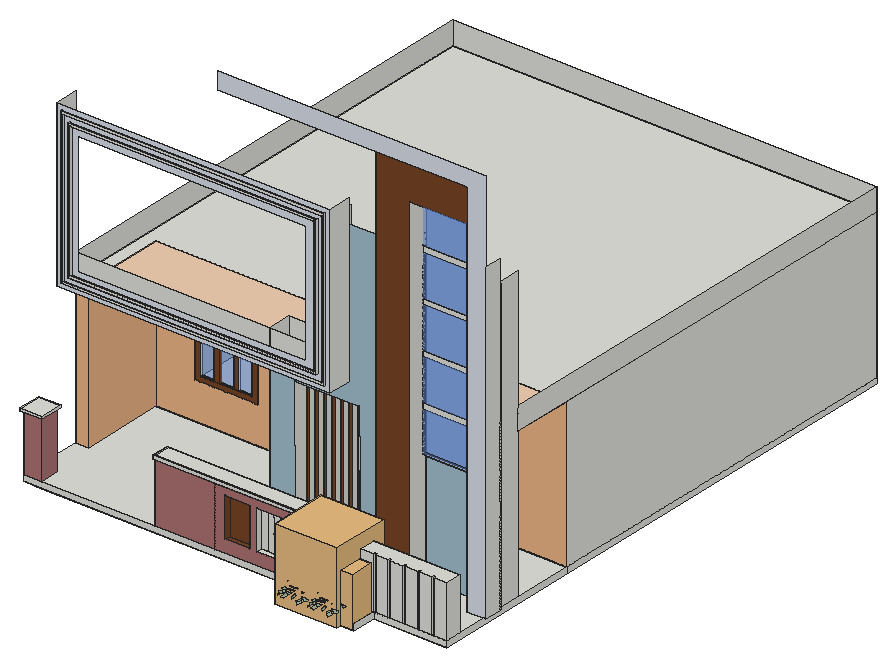
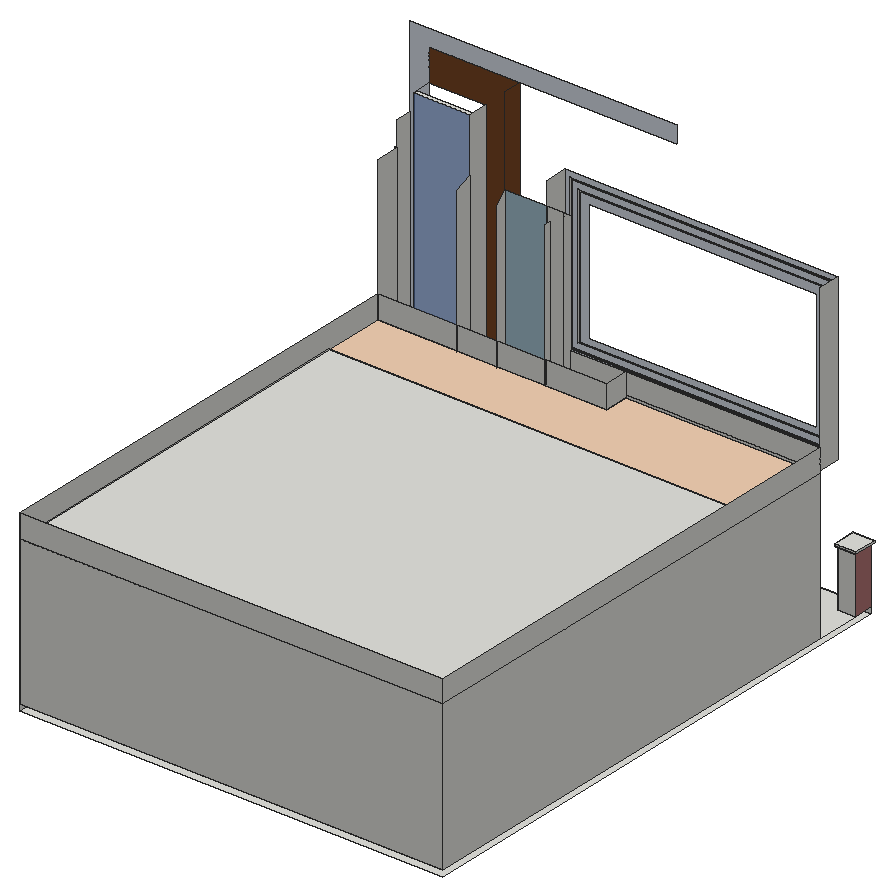
# SketchUp Ruby script. Lengths in inches.
U = 1.inch
M = Sketchup.active_model
def pt(a) = Geom::Point3d.new(a.map { |v| v * U })
def face(e, loops, mat)
  f = e.add_face(loops[0].map { |a| pt(a) })
  loops[1..].each { |l| e.add_face(l.map { |a| pt(a) }).erase! }
  f.material = f.back_material = mat if mat
  f
end
# faces: each face lists its corners as indices into pts; further lists are holes
def faces(e, pts, list, mat = nil) = list.each { |f| face(e, (f[0].is_a?(Array) ? f : [f]).map { |l| l.map { |i| pts[i] } }, mat) }
# xy, xz, yz: faces in a plane at the given z, y or x. An outline is a flat list of corners, or four numbers for a rectangle; further outlines are holes
def ring(l) = l.size == 4 ? [[l[0], l[1]], [l[2], l[1]], [l[2], l[3]], [l[0], l[3]]] : l.each_slice(2).to_a
def flat(e, list, mat, &to3) = list.each { |f| face(e, (f[0].is_a?(Array) ? f : [f]).map { |l| ring(l).map { |u, v| to3.(u, v) } }, mat) }
def xy(e, z, list, mat = nil) = flat(e, list, mat) { |x, y| [x, y, z] }
def xz(e, y, list, mat = nil) = flat(e, list, mat) { |x, z| [x, y, z] }
def yz(e, x, list, mat = nil) = flat(e, list, mat) { |y, z| [x, y, z] }
def lines(e, pts, list) = list.each { |a, b| e.add_line(pt(pts[a]), pt(pts[b])) }
# prism: a flat outline (further loops are holes) pulled along v
def prism(e, loops, v, mat = nil)
  f = face(e, loops, mat); d = Geom::Vector3d.new(v.map { |x| x * U })
  f.pushpull(f.normal.samedirection?(d) ? d.length : -d.length)
end
def box(e, o, s, mat = nil) = prism(e, [[o, [o[0] + s[0], o[1], o[2]], [o[0] + s[0], o[1] + s[1], o[2]], [o[0], o[1] + s[1], o[2]]]], [0, 0, s[2]], mat)
def at(x, y, z, deg = 0) = Geom::Transformation.translation(pt([x, y, z])) * Geom::Transformation.rotation(ORIGIN, Z_AXIS, deg.degrees)
def axes(o, x, y, z) = Geom::Transformation.new([*x, 0, *y, 0, *z, 0, *pt(o).to_a, 1])
def part(name) = M.definitions.add(name)
# library, detail: a bought-in or finely detailed component or shape, given as its bounding box
def library(name, o, s) = part(name).tap { |d| box(d.entities, o, s) }
def detail(e, o, s) = box(e.add_group.entities, o, s)
def put(e, d, t, mat = nil) = e.add_instance(d, t).tap { |i| i.material = mat if mat }
def group(e, t, mat = nil) = e.add_group.tap { |g| g.transformation = t; g.material = mat if mat }.entities
root = M.entities
M.materials.add("Generic").color = [175, 116, 116]
M.materials.add("Generic\#1").color = [243, 208, 179]
M.materials.add("Generic\#2").color = [164, 192, 208]
M.materials.add("Generic\#3").color = [219, 225, 235]
M.materials.add("Generic\#4").color = [240, 183, 136]
M.materials.add("[Translucent Glass Blue]").color = [100, 149, 237]
M.materials["[Translucent Glass Blue]"].alpha = 0.5
M.materials.add("[Wood Veneer 01]").color = [120, 70, 37]
M.materials.add("hymenocallis littoralis").color = [156, 172, 146]
c1 = part("Group\#856")
xy(c1.entities,7.38,[[0,0,5.5,15.91]],"hymenocallis littoralis")
p = [[5.5,28.78,0],[5.5,26.79,3.44],[0,26.79,3.44],[0,28.78,0],[0,23.75,6],[5.5,23.75,6],
  [0,15.91,7.38],[5.5,15.91,7.38]]
faces(c1.entities,p,[[0,1,2,3],[4,2,1,5],[6,4,5,7]],"hymenocallis littoralis")
c2 = part("Group\#854")
xy(c2.entities,7.38,[[0,0,5.5,15.91],[0,15.91,5.5,23.87]],"hymenocallis littoralis")
p = [[5.5,31.07,4.3],[5.5,27.74,6.47],[0,27.74,6.47],[0,31.07,4.3],[0,23.87,7.38],[5.5,23.87,7.38]]
faces(c2.entities,p,[[0,1,2,3],[4,2,1,5]],"hymenocallis littoralis")
c3 = part("Group\#857")
xy(c3.entities,7.38,[[0,0,5.6,15.91]],"hymenocallis littoralis")
p = [[5.6,28.78,0],[5.6,26.79,3.44],[0,26.79,3.44],[0,28.78,0],[0,23.75,6],[5.6,23.75,6],
  [0,15.91,7.38],[5.6,15.91,7.38]]
faces(c3.entities,p,[[0,1,2,3],[4,2,1,5],[6,4,5,7]],"hymenocallis littoralis")
c4 = part("Group\#855")
put(c4.entities,c2,axes([6.09,8.57,-0.52],[0.446,0.85617,0.26089],[-0.18444,-0.19731,0.96283],[0.87582,-0.47754,0.0699]))
put(c4.entities,c2,axes([6.29,7.28,-1.71],[0.37058,0.92707,-0.05667],[-0.32382,0.19004,0.99128],[0.87712,-0.32925,0.34964]))
put(c4.entities,c2,axes([11.04,16.14,-0.7],[1,0,0],[0,0.16628,1.02662],[0,-1.18456,0.19186]))
c5 = part("Group\#860")
put(c5.entities,c1,axes([24.57,32.05,-1.76],[0.9552,-0.22102,-0.19681],[0.4036,0.95545,0.88585],[-0.00568,-0.67859,0.7345]))
put(c5.entities,c1,axes([23.95,29.24,-2.4],[0,1,0],[-0.76041,0,0.64945],[0.64945,0,0.76041]))
put(c5.entities,c1,axes([24.22,24.72,-0.48],[-0.70711,0.70711,0],[-0.32757,-0.32757,0.80237],[0.61237,0.61237,0.5]))
put(c5.entities,c2,axes([20.66,37.22,-0.63],[1.12361,0.03262,0.39091],[-0.43499,0.29739,0.78777],[0.09852,-1.27434,0.37535]))
put(c5.entities,c1,axes([28.75,24.45,-2.4],[-1,0,0],[0,-0.76041,0.64945],[0,0.64945,0.76041]))
put(c5.entities,c3,axes([30.4,30.98,-3.7],[0.65676,-0.72002,0.22414],[0.55667,0.66341,0.5],[-0.50871,-0.20361,0.83652]))
put(c5.entities,c3,axes([32.41,29.61,-3.7],[0.04029,-0.97372,0.22414],[0.85287,0.15038,0.5],[-0.52057,0.17102,0.83652]))
put(c5.entities,c1,axes([31.89,25.85,-1.76],[-0.92056,0.33739,-0.19681],[-0.5186,-0.89824,0.88585],[0.08952,0.67268,0.7345]))
put(c5.entities,c1,axes([25.55,34.78,-0.48],[0.86603,0.5,0],[-0.25,0.43301,0.86603],[0.43301,-0.75,0.5]))
put(c5.entities,c3,axes([20.4,16.9375,-8.07],[-0.70711,0.70711,0],[-0.35754,-0.35754,0.65422],[1.3987,1.3987,1.52882]))
put(c5.entities,c1,axes([32.86,34.14,-0.48],[0.76604,-0.64279,0],[0.32139,0.38302,0.86603],[-0.55667,-0.66341,0.5]))
put(c5.entities,c1,axes([27.15,34.7,-0.1],[0.82472,-0.17528,-0.53769],[0.53769,0.53769,0.64945],[0.17528,-0.82472,0.53769]))
put(c5.entities,c1,axes([33.58,28.77,-2.4],[0,-1,0],[0.76041,0,0.64945],[-0.64945,0,0.76041]))
put(c5.entities,c1,axes([26.43,23.87,-2.81],[-0.75126,0.04415,0.65853],[0.53769,-0.53769,0.64945],[0.38276,0.84199,0.3802]))
put(c5.entities,c1,axes([28.78,23.98,-2.4],[-1,0,0],[0,-0.76041,0.64945],[0,0.64945,0.76041]))
put(c5.entities,c1,axes([25.39,25.38,-2.4],[-0.70711,0.70711,0],[-0.53769,-0.53769,0.64945],[0.45923,0.45923,0.76041]))
put(c5.entities,c1,axes([27.32,21.63,-0.1],[-0.45923,0.70711,-0.53769],[-0.76041,0,0.64945],[0.45923,0.70711,0.53769]))
put(c5.entities,c1,axes([25.17,27.625,-1.76],[0.56416,0.80187,-0.19681],[-0.66673,0.66673,0.80532],[0.62659,-0.26057,0.7345]))
put(c5.entities,c3,axes([27.59,27.04,-3.96],[-0.8993,-0.06127,0.43301],[0.2962,-0.8138,0.5],[0.32175,0.57791,0.75]))
put(c5.entities,c3,axes([26.98,24.5,-3.18],[-0.5,0.86603,0],[-0.75,-0.43301,0.5],[0.43301,0.25,0.86603]))
put(c5.entities,c3,axes([24.55,27.74,-3.7],[0.29517,0.92878,0.22414],[-0.85287,0.15038,0.5],[0.43068,-0.33875,0.83652]))
put(c5.entities,c3,axes([24.26,29.8,-3.18],[0.76604,0.64279,0],[-0.47317,0.5639,0.425],[0.32139,-0.38302,0.86603]))
put(c5.entities,c3,axes([25.98,32.46,-3.18],[1,0,0],[0,0.86603,0.5],[0,-0.5,0.86603]))
put(c5.entities,c1,axes([28.78,33.57,-2.4],[1,0,0],[0,0.76041,0.64945],[0,-0.64945,0.76041]))
put(c5.entities,c4,at(14.99,21.38,2.5))
put(c5.entities,c2,axes([34.63,26.34,-1.46],[-0.70089,-0.70877,0.07994],[0.4756,-0.38088,0.79293],[-0.53156,0.59378,0.60405]))
put(c5.entities,c2,axes([28.14,16.92,1.8125],[-1.19719,0.6912,0],[-0.09607,-0.16641,0.94244],[0.68444,1.18549,0.17613]))
put(c5.entities,c2,axes([31.5625,35.84,0.97],[0.66765,-1.1564,0.35779],[0.04445,0.30732,0.91033],[-1.20828,-0.64496,0.17012]))
put(c5.entities,c2,axes([38.94,22.51,0.89],[-0.97932,-0.67164,-0.05202],[0.27787,-0.41401,0.90999],[-0.85985,0.93577,0.32097]))
put(c5.entities,c2,axes([38.44,21.09,1.98],[-1.02864,-0.54856,0.2395],[0.33481,0.06999,0.88388],[-0.77261,1.08328,0.06417]))
put(c5.entities,c3,axes([35.02,30.51,-1.3],[-0.17365,-0.98481,0],[0.60224,-0.10619,0.79122],[-0.7792,0.13739,0.61153]))
put(c5.entities,c3,axes([29.41,22.33,-1.3],[-0.93969,0.34202,0],[-0.20915,-0.57465,0.79122],[0.27061,0.74351,0.61153]))
put(c5.entities,c2,axes([19.64,36,-1.62],[1.18194,0.09546,0.08234],[-0.14377,0.68823,0.76313],[0.21457,-1.1326,0.62386]))
put(c5.entities,c3,axes([24.25,24.14,-1.3],[-0.34202,0.93969,0],[-0.57465,-0.20915,0.79122],[0.74351,0.27061,0.61153]))
put(c5.entities,c3,axes([25.98,34.61,-1.3],[1,0,0],[0,0.61153,0.79122],[0,-0.79122,0.61153]))
put(c5.entities,c3,axes([31.16,34.41,-1.64],[0.56518,-0.80224,-0.19234],[0.73413,0.34233,0.72935],[-0.47639,-0.50772,0.71782]))
put(c5.entities,c3,axes([40.52,26.84,-5.82],[-0.42262,-0.90631,0],[0.48019,-0.22391,0.68552],[-1.43418,0.66877,1.22305]))
put(c5.entities,c1,axes([29.86,38.42,-1.01],[0.89064,-0.37013,0.26413],[-0.03924,0.63286,1.01918],[-0.45353,-0.76487,0.45748]))
put(c5.entities,c1,axes([29.34,22.4,-0.48],[-0.99619,-0.08716,0],[0.04358,-0.4981,0.86603],[-0.07548,0.86273,0.5]))
c6 = part("Group\#858")
xz(c6.entities,10.07,[[9.07,0,10.07,31.01],[0,31.01,0,45.12,20.13,45.12,20.13,31.01,10.07,31.01,10.07,32.58,9.07,32.58,9.07,31.01]],"hymenocallis littoralis")
yz(c6.entities,10.07,[[0,31.01,20.13,45.12]],"hymenocallis littoralis")
p = [[9.57,9.2,0],[10.07,10.07,0],[10.07,10.07,31.01],[10.07,10.07,32.58],[9.57,9.2,32.58]]
faces(c6.entities,p,[[0,1,2,3,4]],"hymenocallis littoralis")
c7 = part("cây lá nắng")
put(c7.entities,c5,axes([49.26,-2.75,0],[0.63109,0.63109,0],[-0.63109,0.63109,0],[0,0,0.935]))
g1 = group(c7.entities,at(26.6,-8.68,0))
put(g1,c1,axes([-4.72,35.73,-1.65],[0.74231,0.46334,-0.18402],[-0.34827,0.85768,0.82827],[0.42467,-0.43184,0.68675]))
put(g1,c1,axes([-3.34,33.57,-2.24],[-0.63109,0.63109,0],[-0.47989,-0.47989,0.60723],[0.40986,0.40986,0.71098]))
put(g1,c1,axes([-0.3125,30.89,-0.45],[-0.8925,0,0],[0,-0.41345,0.75022],[0,0.77293,0.4675]))
put(g1,c2,axes([-10.79,39.66,-0.59],[0.68852,0.72969,0.3655],[-0.4622,-0.08684,0.73657],[0.86641,-0.74205,0.35095]))
put(g1,c1,axes([2.71,33.57,-2.24],[-0.63109,-0.63109,0],[0.47989,-0.47989,0.60723],[-0.40986,0.40986,0.71098]))
put(g1,c3,axes([-0.37,38.74,-3.46],[0.86887,-0.03992,0.20957],[-0.06737,0.76999,0.4675],[-0.19255,-0.44954,0.78214]))
put(g1,c3,axes([1.76,39.14,-3.46],[0.63993,-0.58908,0.20957],[0.44333,0.63315,0.4675],[-0.43646,-0.2206,0.78214]))
put(g1,c1,axes([3.81,36.4375,-1.65],[-0.79389,-0.36803,-0.18402],[0.23959,-0.89415,0.82827],[-0.36803,0.48102,0.68675]))
put(g1,c1,axes([-5.83,38.07,-0.45],[0.231,0.86209,0],[-0.43104,0.1155,0.80973],[0.74659,-0.20005,0.4675]))
put(g1,c3,axes([2.18,23.5625,-7.55],[-0.8925,0,0],[0,-0.45128,0.6117],[0,1.76542,1.42944]))
put(g1,c1,axes([-0.8125,42.28,-0.45],[0.8891,0.07779,0],[-0.03889,0.44455,0.80973],[0.06737,-0.76999,0.4675]))
put(g1,c1,axes([-4.76,39.03,-0.09],[0.63109,0.40986,-0.50274],[0,0.67866,0.60723],[0.63109,-0.40986,0.50274]))
put(g1,c1,axes([3.03,39.35,-2.24],[0.63109,-0.63109,0],[0.47989,0.47989,0.60723],[-0.40986,-0.40986,0.71098]))
put(g1,c1,axes([1.61,31.74,-2.625],[-0.50198,-0.44625,0.61573],[0.67866,0,0.60723],[-0.28982,0.77293,0.35549]))
put(g1,c1,axes([3.03,33.3,-2.24],[-0.63109,-0.63109,0],[0.47989,-0.47989,0.60723],[-0.40986,0.40986,0.71098]))
put(g1,c1,axes([0.01,32.04,-2.24],[-0.8925,0,0],[0,-0.67866,0.60723],[0,0.57963,0.71098]))
put(g1,c1,axes([3.59,30.89,-0.09],[-0.73607,0.15643,-0.50274],[-0.47989,-0.47989,0.60723],[-0.15643,0.73607,0.50274]))
put(g1,c1,axes([-1.55,33.32,-1.65],[-0.15002,0.86209,-0.18402],[-0.84154,0,0.75297],[0.55988,0.231,0.68675]))
put(g1,c3,axes([0.35,34.48,-3.71],[-0.52887,-0.60621,0.40487],[0.70051,-0.32665,0.4675],[-0.16166,0.56777,0.70125]))
put(g1,c3,axes([2.61,39.13,-1.74],[-0.86209,0.231,0],[-0.23031,-0.85954,0.15531],[0.03162,0.11799,0.91645]))
put(g1,c3,axes([-2.02,33,-3.46],[-0.39986,0.77243,0.20957],[-0.63315,-0.44333,0.4675],[0.48558,0.05802,0.78214]))
put(g1,c3,axes([-3.49,34.12,-2.97],[0.07779,0.8891,0],[-0.65449,0.05726,0.39737],[0.44455,-0.03889,0.80973]))
put(g1,c3,axes([-4.09,36.88,-2.97],[0.63109,0.63109,0],[-0.54654,0.54654,0.4675],[0.31555,-0.31555,0.80973]))
put(g1,c1,axes([-3.02,39.35,-2.24],[0.63109,0.63109,0],[-0.47989,0.47989,0.60723],[0.40986,-0.40986,0.71098]))
put(g1,c4,axes([-4.03,22.95,2.33],[0.63109,0.63109,0],[-0.63109,0.63109,0],[0,0,0.935]))
put(g1,c2,axes([5.24,38.48,-1.37],[0.00497,-0.88963,0.07474],[0.54052,0.05978,0.74139],[-0.71019,0.03927,0.56479]))
put(g1,c2,axes([7.08,28.4375,1.7],[-1.19175,-0.31933,0],[0.04439,-0.16565,0.88118],[-0.31621,1.1801,0.16468]))
put(g1,c2,axes([-2.7,42.54,0.91],[1.15114,-0.30845,0.33454],[-0.1659,0.22199,0.85115],[-0.3555,-1.16957,0.15907]))
put(g1,c2,axes([10.37,38.78,0.83],[-0.19417,-1.04191,-0.04864],[0.43664,-0.08592,0.85084],[-1.1332,0.04791,0.30011]))
put(g1,c2,axes([10.95,37.5625,1.85],[-0.30298,-0.99536,0.22393],[0.16713,0.25547,0.82643],[-1.17124,0.19607,0.06]))
put(g1,c3,axes([2.84,41.36,-1.22],[0.51192,-0.73109,0],[0.44708,0.31305,0.73979],[-0.57846,-0.40504,0.57178]))
put(g1,c3,axes([4.47,32.65,-1.22],[-0.80888,-0.37719,0],[0.23066,-0.49465,0.73979],[-0.29844,0.64,0.57178]))
put(g1,c2,axes([-10.32,35.12,-1.51],[0.68567,0.80616,0.07699],[-0.52507,0.3436,0.71352],[0.85019,-0.57936,0.58331]))
put(g1,c3,axes([0.07,30.54,-1.22],[-0.80888,0.37719,0],[-0.23066,-0.49465,0.73979],[0.29844,0.64,0.57178]))
put(g1,c3,axes([-5.45,38.24,-1.22],[0.63109,0.63109,0],[-0.38593,0.38593,0.73979],[0.49934,-0.49934,0.57178]))
put(g1,c3,axes([-2.05,41.38,-1.53],[0.86296,-0.14961,-0.17984],[0.24726,0.67935,0.68194],[0.01977,-0.62107,0.67116]))
put(g1,c3,axes([8.63,42.51,-5.4375],[0.30525,-0.83868,0],[0.44435,0.16173,0.64096],[-1.32716,-0.48305,1.14356]))
put(g1,c1,axes([-5.4,43.09,-0.94],[0.79566,0.32849,0.24696],[-0.42416,0.37462,0.95293],[0.19648,-0.76892,0.42774]))
put(g1,c1,axes([4.38,32.65,-0.45],[-0.57369,-0.68369,0],[0.34185,-0.28684,0.80973],[-0.5921,0.49683,0.4675]))
put(g1,c3,axes([-2,33.84,-0.15],[-0.24601,0.85793,0],[-0.85539,-0.24528,0.15531],[0.11742,0.03367,0.91645]))
put(g1,c3,axes([0.17,30.83,-4.47],[-0.24601,0.85793,0],[-0.85539,-0.24528,0.15531],[0.11742,0.03367,0.91645]))
put(g1,c3,axes([-1.97,32.18,-4.47],[0.58524,0.67383,0],[-0.67184,0.58351,0.15531],[0.09222,-0.0801,0.91645]))
put(g1,c3,axes([-2,34.71,-4.47],[0.88392,-0.12346,0],[0.12309,0.88131,0.15531],[-0.0169,-0.12098,0.91645]))
put(g1,c3,axes([0.11,36.12,-4.47],[0.37822,-0.8084,0],[0.80601,0.37711,0.15531],[-0.11064,-0.05177,0.91645]))
put(c7.entities,c6,axes([29.71,14.29,6.94],[0.425,0.73612,0],[-0.6771,0.39092,-0.33349],[-0.26859,0.15507,0.72712]))
put(c7.entities,c6,axes([42.0625,26.12,6.94],[0.85,0,0],[0,0.78185,-0.33349],[0,0.33349,0.78185]))
put(c7.entities,c5,axes([7.3125,23.0625,0],[0.8925,0,0],[0,0.8925,0],[0,0,0.935]))
put(c7.entities,c6,axes([24.4375,40.23,2.05],[0.85,0,0],[0,0.85,0],[0,0,0.85]))
c8 = part("Planting+101")
put(c8.entities,c7,axes([21.34,32.96,-4.59],[0,-0.71,0],[-0.71,0,0],[0,0,0.71]))
c9 = library("Flora+17",[-57.52,158.6,-38.64],[66.99,62.88,77.28])
c10 = library("Group38\#2",[14.01,28.44,-23.43],[18.58,18.32,38.89])
c11 = library("Group\#4",[0,0,0],[42.5625,8.58,93.9375])
xy(root,-33.1875,[[283,11.84,283,36.4,15.9375,36.4,15.9375,184.78,423.0625,184.78,423.0625,36.4,350.18,36.4,350.18,11.84],[3.0625,36.4,3.0625,568.65,423.0625,568.65,423.0625,184.78,15.9375,184.78,15.9375,36.4]])
xy(root,-33,[[286.34,15.18,346.84,33.07]])
xy(root,-27.1875,[[[283,11.84,350.18,36.4],[286.34,15.18,346.84,33.07]],[20.96,36.4,133.46,36.4,133.46,52.83,423.0625,52.83,423.0625,81.53,406.3,81.53,406.3,100.72,350.4375,100.72,350.4375,81.53,316,81.53,316,100.72,195.4375,100.72,195.4375,124.65,423.0625,124.65,423.0625,184.78,15.9375,184.78,15.9375,100.72,3.0625,100.72,3.0625,55.77,20.96,55.77],[3.0625,36.4,20.96,55.77],[133.46,36.4,133.46,52.83,423.0625,52.83,423.0625,36.4,409.92,36.4,409.92,38.28,408.49,38.28,408.49,36.4,395.35,36.4,395.35,38.28,393.91,38.28,393.91,36.4,380.77,36.4,380.77,38.28,379.33,38.28,379.33,36.4,366.2,36.4,366.2,38.28,364.76,38.28,364.76,36.4,352,36.4,352,38.28,350.18,38.28,350.18,36.4],[350.18,36.4,352,38.28],
  [364.76,36.4,366.2,38.28],[379.33,36.4,380.77,38.28],[393.91,36.4,395.35,38.28],[408.49,36.4,409.92,38.28],[316,81.53,350.4375,81.53,350.4375,100.72,344.25,124.65,304.375,124.65,316,100.72],
  [406.3,81.53,423.0625,100.72],[423.0625,81.53,425.125,100.72],[3.0625,100.72,15.9375,100.72,15.9375,184.78,423.0625,184.78,423.0625,568.65,3.0625,568.65],[195.4375,100.72,316,100.72,304.375,124.65,195.4375,124.65],[350.4375,100.72,423.0625,100.72,423.0625,124.65,344.25,124.65]])
xy(root,-14.28,[[234.3125,36.4,272.75,41.84]])
xy(root,-14.28,[[202.9375,36.4,227.1875,41.84]],"[Wood Veneer 01]")
xy(root,-12.24,[[148.15,184.78,190.71,360.72]])
xy(root,-9.79,[[[221.76,100.72,285.14,124.65],[275.89,109.625,279.51,116.52],[267.45,109.625,271.08,116.52],[259.01,109.625,262.64,116.52],[250.58,109.625,254.2,116.52],[242.14,109.625,245.76,116.52],[233.7,109.625,237.33,116.52],[225.26,109.625,228.89,116.52]],[285.14,109.625,287.95,116.52],[292.76,109.625,296.39,116.52]])
xy(root,9.62,[[54.62,184.78,116.37,362.97]])
xy(root,24.0625,[[283,36.4,350.18,36.4,350.18,38.28,352,38.28,352,36.4,364.76,36.4,364.76,38.28,366.2,38.28,366.2,36.4,379.33,36.4,379.33,38.28,380.77,38.28,380.77,36.4,393.91,36.4,393.91,38.28,395.35,38.28,395.35,36.4,408.49,36.4,408.49,38.28,409.92,38.28,409.92,36.4,423.0625,36.4,423.0625,52.83,284.33,52.83,284.33,49.39]])
xy(root,24.66,[[234.3125,36.4,272.75,41.84]])
xy(root,24.66,[[202.9375,36.4,227.1875,41.84]],"[Wood Veneer 01]")
xy(root,29.8125,[[1.3125,34.65,22.71,36.4],[1.3125,36.4,3.0625,57.52],[3.0625,36.4,20.96,55.77],[20.96,36.4,22.71,57.52],[3.0625,55.77,20.96,57.52]])
xy(root,31.9375,[[1.3125,34.65,22.71,57.52]])
xy(root,33.125,[[132.09,35.03,133.46,36.4],[133.46,35.03,193.21,36.4],[193.21,35.03,283,36.4],[132.09,36.4,133.46,52.83]])
xy(root,35.9375,[[132.09,35.03,283,35.03,283,36.4,133.46,36.4,133.46,52.83,132.09,52.83],[133.46,36.4,283,36.4,284.33,49.39,284.33,52.83,133.46,52.83]])
xy(root,74.93,[[54.62,184.78,116.37,362.97]])
xy(root,81.69,[[148.15,184.78,190.71,360.72]])
xy(root,103.27,[[225.26,109.625,228.89,116.52],[233.7,109.625,237.33,116.52],[242.14,109.625,245.76,116.52],[250.58,109.625,254.2,116.52],[259.01,109.625,262.64,116.52],
  [267.45,109.625,271.08,116.52],[275.89,109.625,279.51,116.52]])
xy(root,104.16,[[230.83,100.72,284.52,124.65]])
xy(root,120,[[3.0625,100.72,3.0625,568.65,423.0625,568.65,423.0625,184.78,15.9375,184.78,15.9375,100.72],[195.4375,118.03,257,124.65]])
xy(root,120,[[15.9375,100.72,15.9375,184.78,423.0625,184.78,423.0625,124.65,195.4375,124.65,195.4375,100.72]],"Generic\#1")
xy(root,122.375,[[3.0625,77.59,274.375,100.72]])
xy(root,127.37,[[8.06,75.97,269.38,77.59]])
xy(root,129.45,[[10.13,75.97,267.3,77.59]])
xy(root,135.08,[[15.77,75.97,261.67,77.59]])
xy(root,137.125,[[17.8125,75.97,259.625,77.59]])
xz(root,11.84,[[283,-33.1875,350.18,-27.1875]])
xz(root,15.18,[[286.34,-33,346.84,-27.1875]])
xz(root,33.07,[[286.34,-33,346.84,-27.1875]])
xz(root,34.65,[[1.3125,29.8125,22.71,31.9375]])
xz(root,35.03,[[132.09,33.125,283,35.9375]])
xz(root,36.4,[[3.0625,-33.1875,283,-27.1875],[350.18,-33.1875,423.0625,-27.1875],[283,-27.1875,350.18,24.0625],[352,-27.1875,364.76,24.0625],[366.2,-27.1875,379.33,24.0625],
  [380.77,-27.1875,393.91,24.0625],[395.35,-27.1875,408.49,24.0625],[409.92,-27.1875,423.0625,24.0625],[133.46,33.125,283,35.9375]])
xz(root,36.4,[[3.0625,-27.1875,20.96,29.8125],[133.46,-27.1875,193.21,33.125],[[193.21,-27.1875,283,33.125],[234.3125,-14.28,272.75,24.66],[202.9375,-14.28,227.1875,24.66]]],"Generic")
xz(root,38.28,[[350.18,-27.1875,352,24.0625],[364.76,-27.1875,366.2,24.0625],[379.33,-27.1875,380.77,24.0625],[393.91,-27.1875,395.35,24.0625],[408.49,-27.1875,409.92,24.0625]])
xz(root,41.84,[[234.3125,-14.28,240.72,24.66],[240.72,-14.28,247.125,24.66],[247.125,-14.28,253.53,24.66],[253.53,-14.28,259.9375,24.66],[259.9375,-14.28,266.34,24.66],
  [266.34,-14.28,272.75,24.66]])
xz(root,41.84,[[202.9375,-14.28,227.1875,24.66]],"[Wood Veneer 01]")
xz(root,52.83,[[133.46,-27.1875,133.46,35.9375,284.33,35.9375,284.33,24.0625,423.0625,24.0625,423.0625,-27.1875],[132.09,33.125,133.46,35.9375]])
xz(root,55.77,[[3.0625,-27.1875,20.96,29.8125]])
xz(root,57.52,[[1.3125,29.8125,22.71,31.9375]])
xz(root,75.97,[[[8.06,127.37,269.38,280.38],[10.13,129.45,267.3,278.3]],[[15.77,135.08,261.67,272.67],[17.8125,137.125,259.625,270.625]]])
xz(root,77.59,[[[3.0625,122.375,274.375,285.375],[8.06,127.37,269.38,280.38]],[[10.13,129.45,267.3,278.3],[15.77,135.08,261.67,272.67]],[[17.8125,137.125,259.625,270.625],[24.3125,142.6875,250.5625,262.6875]]],"Generic\#3")
xz(root,81.53,[[406.3,-27.1875,425.125,-27.1875,425.125,366.8125,160.125,366.8125,160.125,349.9375,406.3,349.9375]],"Generic\#3")
xz(root,81.53,[[316,-27.1875,350.4375,-27.1875,350.4375,317.5625,406.3,317.5625,406.3,349.9375,316,349.9375]],"[Wood Veneer 01]")
xz(root,100.72,[[423.0625,-27.1875,425.125,262.6875],[350.4375,85.625,406.3,317.5625],[3.0625,120,195.4375,122.375],[3.0625,122.375,195.4375,142.6875],[195.4375,122.375,250.5625,142.6875],
  [250.5625,122.375,257,262.6875],[257,122.375,274.375,262.6875]])
xz(root,100.72,[[[195.4375,-27.1875,316,-27.1875,316,262.6875,274.375,262.6875,274.375,122.375,195.4375,122.375],[221.76,-9.79,221.14,104.11,230.83,104.16,284.52,104.16,285.14,-9.79]],[350.4375,-27.1875,406.3,85.625]],"Generic\#2")
xz(root,100.72,[[3.0625,-27.1875,15.9375,120]],"Generic\#4")
xz(root,109.625,[[225.26,-9.79,228.89,103.27],[233.7,-9.79,237.33,103.27],[242.14,-9.79,245.76,103.27],[250.58,-9.79,254.2,103.27],[259.01,-9.79,262.64,103.27],
  [267.45,-9.79,271.08,103.27],[275.89,-9.79,279.51,103.27]],"[Wood Veneer 01]")
xz(root,116.52,[[225.26,-9.79,228.89,103.27]])
xz(root,116.52,[[233.7,-9.79,237.33,103.27],[242.14,-9.79,245.76,103.27],[250.58,-9.79,254.2,103.27],[259.01,-9.79,262.64,103.27],[267.45,-9.79,271.08,103.27],
  [275.89,-9.79,279.51,103.27]],"[Wood Veneer 01]")
xz(root,124.65,[[[195.4375,-27.1875,304.375,120],[221.76,-9.79,221.14,104.11,230.83,104.16,284.52,104.16,285.14,-9.79]],[304.375,-27.1875,344.25,120],[344.25,-27.1875,423.0625,120],[195.4375,120,256.02,142.6875],[256.02,120,257,142.6875],
  [257,120,304.375,142.6875],[304.375,120,344.25,142.6875],[344.25,120,423.0625,142.6875]])
xz(root,184.78,[[15.9375,-33.1875,423.0625,-27.1875]])
xz(root,184.78,[[[15.9375,-27.1875,423.0625,120],[54.62,9.62,116.37,74.93],[148.15,-12.24,190.71,81.69]]],"Generic\#4")
xz(root,360.72,[[148.15,-12.24,190.71,81.69]])
xz(root,362.97,[[54.62,9.62,116.37,74.93]])
xz(root,568.65,[[3.0625,-27.1875,423.0625,120],[3.0625,120,423.0625,142.6875]])
yz(root,1.3125,[[34.65,29.8125,57.52,31.9375]])
yz(root,3.0625,[[100.72,-27.1875,568.65,120],[100.72,120,568.65,142.6875],[77.59,122.375,100.72,285.375]])
yz(root,3.0625,[[36.4,-27.1875,55.77,29.8125]],"Generic")
yz(root,8.06,[[75.97,127.37,77.59,280.38]])
yz(root,10.13,[[75.97,129.45,77.59,278.3]])
yz(root,15.77,[[75.97,135.08,77.59,272.67]])
yz(root,15.9375,[[100.72,-27.1875,184.78,120]],"Generic\#4")
yz(root,17.8125,[[75.97,137.125,77.59,270.625]])
yz(root,20.96,[[36.4,-27.1875,55.77,29.8125]],"Generic")
yz(root,22.71,[[34.65,29.8125,57.52,31.9375]])
yz(root,54.62,[[184.78,9.62,362.97,74.93]])
yz(root,116.37,[[184.78,9.62,362.97,74.93]])
yz(root,132.09,[[35.03,33.125,52.83,35.9375]])
yz(root,133.46,[[36.4,-27.1875,52.83,33.125],[36.4,33.125,52.83,35.9375]])
yz(root,148.15,[[184.78,-12.24,360.72,81.69]])
yz(root,190.71,[[184.78,-12.24,360.72,81.69]])
yz(root,195.4375,[[100.72,-27.1875,124.65,120],[100.72,120,124.65,142.6875]])
yz(root,202.9375,[[36.4,-14.28,41.84,24.66]],"[Wood Veneer 01]")
yz(root,221.76,[[100.72,-9.85,124.65,-9.79]])
yz(root,225.26,[[109.625,-9.79,116.52,103.27]],"[Wood Veneer 01]")
yz(root,227.1875,[[36.4,-14.28,41.84,24.66]],"[Wood Veneer 01]")
yz(root,228.89,[[109.625,-9.79,116.52,103.27]])
yz(root,233.7,[[109.625,-9.79,116.52,103.27]],"[Wood Veneer 01]")
yz(root,234.3125,[[36.4,-14.28,41.84,24.66]])
yz(root,237.33,[[109.625,-9.79,116.52,103.27]])
yz(root,242.14,[[109.625,-9.79,116.52,103.27]],"[Wood Veneer 01]")
yz(root,245.76,[[109.625,-9.79,116.52,103.27]])
yz(root,250.58,[[109.625,-9.79,116.52,103.27]],"[Wood Veneer 01]")
yz(root,254.2,[[109.625,-9.79,116.52,103.27]])
yz(root,257,[[118.03,120,124.65,262.6875]])
yz(root,259.01,[[109.625,-9.79,116.52,103.27]],"[Wood Veneer 01]")
yz(root,259.625,[[75.97,137.125,77.59,270.625]])
yz(root,261.67,[[75.97,135.08,77.59,272.67]])
yz(root,262.64,[[109.625,-9.79,116.52,103.27]])
yz(root,267.3,[[75.97,129.45,77.59,278.3]])
yz(root,267.45,[[109.625,-9.79,116.52,103.27]],"[Wood Veneer 01]")
yz(root,269.38,[[75.97,127.37,77.59,280.38]])
yz(root,271.08,[[109.625,-9.79,116.52,103.27]])
yz(root,272.75,[[36.4,-14.28,41.84,24.66]])
yz(root,274.375,[[77.59,122.375,100.72,285.375]])
yz(root,275.89,[[109.625,-9.79,116.52,103.27]],"[Wood Veneer 01]")
yz(root,279.51,[[109.625,-9.79,116.52,103.27]])
yz(root,283,[[11.84,-33.1875,36.4,-27.1875],[35.03,33.125,36.4,35.9375]])
yz(root,284.33,[[49.39,24.0625,52.83,35.9375]])
yz(root,286.34,[[15.18,-33,33.07,-27.1875]])
yz(root,316,[[81.53,-27.1875,100.72,349.9375]],"[Wood Veneer 01]")
yz(root,346.84,[[15.18,-33,33.07,-27.1875]])
yz(root,350.18,[[11.84,-33.1875,36.4,-27.1875],[36.4,-27.1875,38.28,24.0625]])
yz(root,350.4375,[[81.53,-27.1875,100.72,317.5625]])
yz(root,352,[[36.4,-27.1875,38.28,24.0625]])
yz(root,364.76,[[36.4,-27.1875,38.28,24.0625]])
yz(root,366.2,[[36.4,-27.1875,38.28,24.0625]])
yz(root,379.33,[[36.4,-27.1875,38.28,24.0625]])
yz(root,380.77,[[36.4,-27.1875,38.28,24.0625]])
yz(root,393.91,[[36.4,-27.1875,38.28,24.0625]])
yz(root,395.35,[[36.4,-27.1875,38.28,24.0625]])
yz(root,406.3,[[81.53,-27.1875,100.72,317.5625]],"Generic\#3")
yz(root,408.49,[[36.4,-27.1875,38.28,24.0625]])
yz(root,409.92,[[36.4,-27.1875,38.28,24.0625]])
yz(root,423.0625,[[36.4,-33.1875,184.78,-27.1875],[184.78,-33.1875,568.65,-27.1875],[36.4,-27.1875,52.83,24.0625],[100.72,-27.1875,124.65,262.6875],[184.78,-27.1875,568.65,120],
  [124.65,120,568.65,142.6875]])
yz(root,425.125,[[81.53,-27.1875,98.72,285.375],[98.72,-27.1875,100.72,142.6875]])
p = [[316,100.72,262.6875],[316,100.72,-27.1875],[304.375,124.65,-27.1875],[304.375,124.65,120],[304.375,124.65,142.6875],[304.375,124.65,262.6875],
  [344.25,124.65,262.6875],[344.25,124.65,142.6875],[344.25,124.65,120],[344.25,124.65,-27.1875],[350.4375,100.72,-27.1875],[350.4375,100.72,85.625],
  [350.4375,100.72,262.6875],[221.14,124.65,104.11],[221.14,100.72,104.11],[221.76,100.72,-9.79],[221.76,124.65,-9.79],[285.14,109.625,-9.79],
  [285.14,100.72,-9.79],[284.52,100.72,104.16],[284.52,124.65,104.16],[285.14,124.65,-9.79],[285.14,116.52,-9.79],[284.33,49.39,35.9375],
  [283,36.4,35.9375],[283,36.4,33.125],[283,36.4,24.0625],[284.33,49.39,24.0625],[230.83,124.65,104.16],[230.83,100.72,104.16],
  [257,118.03,120],[257,100.72,120]]
faces(root,p,[[0,1,2,3,4,5],[6,7,8,9,10,11,12],[13,14,15,16],[17,18,19,20,21,22],[23,24,25,26,27],[28,29,14,13]])
lines(root,p,[[30,31]])
put(root,c8,at(296.75,18.4375,-25.07))
put(root,c8,at(326.68,18.4375,-25.07))
put(root,c9,axes([328.01,-138.28,1.75],[0.92,0,0],[0,0.92,0],[0,0,0.92]))
put(root,c10,axes([307.71,-24.16,-3.53],[1.2656,0,0],[0,1.2656,0],[0,0,1.2656]))
put(root,c11,at(148.15,182.39,-12.24))
g2 = group(root,at(54.62,184.78,9.62))
xy(g2,0,[[0,0,61.75,2.3125]])
xy(g2,5.1875,[[37.71,0.625,42.9,2.3125]])
xy(g2,5.1875,[[5.1875,0,18.85,2.3125],[18.85,0,24.04,2.3125],[24.04,0,37.71,2.3125],[37.71,0,42.9,0.625],[42.9,0,56.5625,2.3125]],"[Wood Veneer 01]")
xy(g2,60.125,[[5.1875,0,18.85,2.3125],[18.85,0,24.04,2.3125],[24.04,0,37.71,2.3125],[37.71,0,42.9,0.625],[42.9,0,56.5625,2.3125],
  [37.71,0.625,42.9,2.3125]])
xy(g2,65.3125,[[0,0,61.75,2.3125]],"[Wood Veneer 01]")
xz(g2,0,[[[0,0,61.75,65.3125],[5.1875,5.1875,56.5625,60.125]],[18.85,5.1875,24.04,60.125]],"[Wood Veneer 01]")
xz(g2,0.625,[[37.71,5.1875,42.9,60.125]],"[Wood Veneer 01]")
xz(g2,2.3125,[[5.1875,5.1875,18.85,60.125],[24.04,5.1875,37.71,60.125],[42.9,5.1875,56.5625,60.125]],"[Translucent Glass Blue]")
xz(g2,2.3125,[[[0,0,61.75,65.3125],[5.1875,5.1875,56.5625,60.125]]],"[Wood Veneer 01]")
yz(g2,0,[[0,0,2.3125,65.3125]],"[Wood Veneer 01]")
yz(g2,5.1875,[[0,5.1875,2.3125,60.125]])
yz(g2,18.85,[[0,5.1875,2.3125,60.125]],"[Wood Veneer 01]")
yz(g2,24.04,[[0,5.1875,2.3125,60.125]],"[Wood Veneer 01]")
yz(g2,37.71,[[0.625,5.1875,2.3125,60.125]],"[Wood Veneer 01]")
yz(g2,42.9,[[0.625,5.1875,2.3125,60.125]])
yz(g2,56.5625,[[0,5.1875,2.3125,60.125]],"[Wood Veneer 01]")
yz(g2,61.75,[[0,0,2.3125,65.3125]],"[Wood Veneer 01]")
g3 = group(root,at(350.4375,96.78,85.625))
xy(g3,0,[[0,0,55.86,3.9375]])
xy(g3,231.9375,[[0,0,55.86,3.9375]])
xz(g3,0,[[0,41.39,55.86,46.39],[0,87.77,55.86,92.77],[0,134.16,55.86,139.16],[0,180.55,55.86,185.55]])
xz(g3,0,[[0,0,55.86,41.39],[0,46.39,55.86,87.77],[0,92.77,55.86,134.16],[0,139.16,55.86,180.55],[0,185.55,55.86,231.9375]],"[Translucent Glass Blue]")
xz(g3,3.9375,[[0,0,55.86,231.9375]],"[Translucent Glass Blue]")
yz(g3,0,[[0,0,3.9375,177.0625],[0,177.0625,3.9375,199.75],[0,199.75,3.9375,231.9375]])
yz(g3,55.86,[[0,0,3.9375,231.9375]])
